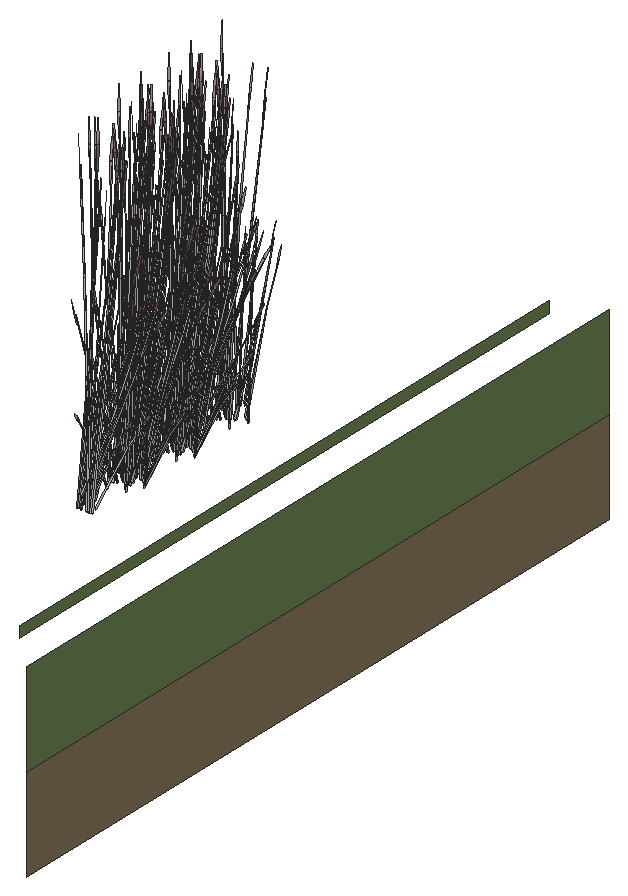
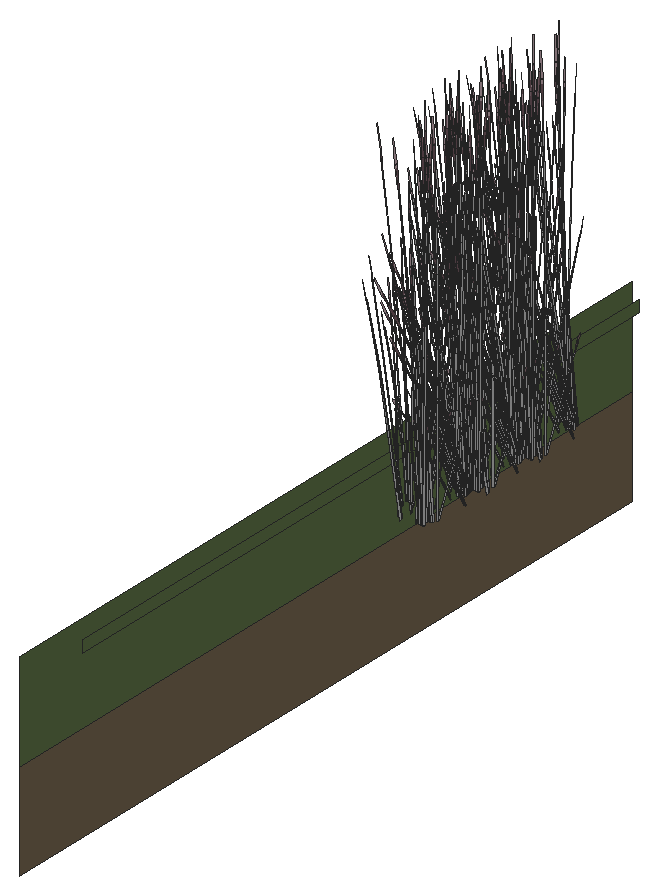
# SketchUp Ruby script. Lengths in inches.
U = 1.inch
M = Sketchup.active_model
def pt(a) = Geom::Point3d.new(a.map { |v| v * U })
def face(e, loops, mat)
  f = e.add_face(loops[0].map { |a| pt(a) })
  loops[1..].each { |l| e.add_face(l.map { |a| pt(a) }).erase! }
  f.material = f.back_material = mat if mat
  f
end
# faces: each face lists its corners as indices into pts; further lists are holes
def faces(e, pts, list, mat = nil) = list.each { |f| face(e, (f[0].is_a?(Array) ? f : [f]).map { |l| l.map { |i| pts[i] } }, mat) }
# xy, xz, yz: faces in a plane at the given z, y or x. An outline is a flat list of corners, or four numbers for a rectangle; further outlines are holes
def ring(l) = l.size == 4 ? [[l[0], l[1]], [l[2], l[1]], [l[2], l[3]], [l[0], l[3]]] : l.each_slice(2).to_a
def flat(e, list, mat, &to3) = list.each { |f| face(e, (f[0].is_a?(Array) ? f : [f]).map { |l| ring(l).map { |u, v| to3.(u, v) } }, mat) }
def xy(e, z, list, mat = nil) = flat(e, list, mat) { |x, y| [x, y, z] }
def xz(e, y, list, mat = nil) = flat(e, list, mat) { |x, z| [x, y, z] }
def yz(e, x, list, mat = nil) = flat(e, list, mat) { |y, z| [x, y, z] }
def lines(e, pts, list) = list.each { |a, b| e.add_line(pt(pts[a]), pt(pts[b])) }
# prism: a flat outline (further loops are holes) pulled along v
def prism(e, loops, v, mat = nil)
  f = face(e, loops, mat); d = Geom::Vector3d.new(v.map { |x| x * U })
  f.pushpull(f.normal.samedirection?(d) ? d.length : -d.length)
end
def box(e, o, s, mat = nil) = prism(e, [[o, [o[0] + s[0], o[1], o[2]], [o[0] + s[0], o[1] + s[1], o[2]], [o[0], o[1] + s[1], o[2]]]], [0, 0, s[2]], mat)
def at(x, y, z, deg = 0) = Geom::Transformation.translation(pt([x, y, z])) * Geom::Transformation.rotation(ORIGIN, Z_AXIS, deg.degrees)
def axes(o, x, y, z) = Geom::Transformation.new([*x, 0, *y, 0, *z, 0, *pt(o).to_a, 1])
def part(name) = M.definitions.add(name)
# library, detail: a bought-in or finely detailed component or shape, given as its bounding box
def library(name, o, s) = part(name).tap { |d| box(d.entities, o, s) }
def detail(e, o, s) = box(e.add_group.entities, o, s)
def put(e, d, t, mat = nil) = e.add_instance(d, t).tap { |i| i.material = mat if mat }
def group(e, t, mat = nil) = e.add_group.tap { |g| g.transformation = t; g.material = mat if mat }.entities
root = M.entities
M.materials.add("LightPink_Translucent").color = [144, 107, 117]
M.materials["LightPink_Translucent"].alpha = 0.75
M.materials.add("Plaster_03_1K").color = [121, 105, 83]
M.materials.add("Roofing_02_1K").color = [97, 118, 74]
M.materials.add("[_0053_Ivory_]").color = [200, 200, 200]
c1 = part("blade")
p = [[2.15,0.21,22],[0,0.17,0],[0.09,0.45,0],[2.18,0.31,22],[2.29,0.31,22],[0.38,0.45,0],
  [2.48,0.24,33],[2.49,0.24,33],[2.48,0.22,33]]
faces(c1.entities,p,[[0,1,2,3],[4,5,2,3],[6,3,4,7],[8,0,3,6]])
c2 = part("seeds")
p = [[0.3,-0.1,1.38],[-0.01,-0.03,1.59],[-0.01,-0.03,0.03],[0.14,-0.07,-0.07],[0.29,-0.03,3],[0.15,0.01,3.11]]
faces(c2.entities,p,[[0,1,2,3],[1,0,4,5]],"LightPink_Translucent")
c3 = part("blade with seeds")
put(c3.entities,c1,at(0,0,0))
put(c3.entities,c2,axes([2.4,0.25,30.99],[1.5799,-0.05474,1.17369],[-0.12525,1.92788,0.29478],[-0.07173,-0.02425,1.56792]))
yz(root,695.51,[[245.15,34,365.15,36]],"Roofing_02_1K")
yz(root,701.51,[[239.15,0,371.15,17]],"Plaster_03_1K")
yz(root,701.51,[[239.15,17,371.15,34]],"Roofing_02_1K")
put(root,c3,axes([680.55,278.33,35.86],[0.61229,0.28233,0],[-0.29468,0.58663,0],[0,0,1.74954]),"[_0053_Ivory_]")
put(root,c3,axes([681.82,278.08,38.63],[0.60713,0.01514,-0.71045],[-0.04078,0.63759,0.08574],[0.25721,0.06729,1.00501]),"[_0053_Ivory_]")
put(root,c3,axes([681.13,278.59,36.13],[0.56842,-0.31443,0.49651],[0.33976,0.56381,0],[-0.12946,0.07161,1.57504]),"[_0053_Ivory_]")
put(root,c3,axes([680.32,278.09,35.94],[0.26406,0.72244,-0.06012],[-0.7545,0.25315,0],[0.00922,0.02523,1.72173]),"[_0053_Ivory_]")
put(root,c3,axes([682.81,276.78,36.03],[0.75945,0,0],[0,0.70283,-0.51607],[0,0.16007,1.63711]),"[_0053_Ivory_]")
put(root,c3,axes([682.51,277.14,35.85],[-0.75908,-0.00503,-0.04976],[0,-0.70283,0.49943],[-0.02386,0.16,1.58352]),"[_0053_Ivory_]")
put(root,c3,axes([680.86,276.53,36.32],[0.68399,0.30005,-0.29095],[-0.32934,0.63331,-0.50002],[0.0215,0.15549,1.59708]),"[_0053_Ivory_]")
put(root,c3,axes([682.18,278.34,38.18],[0.34557,0.39372,-0.35414],[-0.39459,0.37271,0.4572],[0.20048,0.05671,0.87481]),"[_0053_Ivory_]")
put(root,c3,axes([682.35,277.25,35.68],[-0.42396,0.39235,-0.30978],[-0.42396,-0.39235,0.30978],[0,0.12637,1.38974]),"[_0053_Ivory_]")
put(root,c3,axes([680.79,277,35.86],[-0.29468,0.56664,-0.44739],[-0.61229,-0.27271,0.21531],[0,0.13062,1.43643]),"[_0053_Ivory_]")
put(root,c3,axes([680.81,278.63,35.98],[0.76036,0.2044,0.30756],[-0.19023,0.7306,-0.36492],[-0.12585,0.09144,1.64885]),"[_0053_Ivory_]")
put(root,c3,axes([682.64,277.26,35.67],[0,0.62885,-0.49651],[-0.67951,0,0],[0,0.14322,1.57504]),"[_0053_Ivory_]")
put(root,c3,axes([680.94,277.33,37.53],[-0.2256,-0.10835,1.71376],[0.46687,-0.45453,0.13857],[0.29098,0.20505,0.73262]),"[_0053_Ivory_]")
put(root,c3,axes([680.98,285.76,36.24],[-0.17264,0.12729,1.43002],[-0.51703,-0.22279,-0.30754],[0.09584,-0.27707,0.61141]),"[_0053_Ivory_]")
put(root,c3,axes([681.78,278.5625,36.42],[-0.34197,-0.18082,1.1486],[0.44156,-0.18372,0.84392],[0.1191,0.15563,0.25299]),"[_0053_Ivory_]")
put(root,c3,axes([679.7,285.07,35.15],[-0.10187,0.02266,1.76342],[-0.56336,-0.25503,-0.26939],[0.00945,-0.21273,0.30037]),"[_0053_Ivory_]")
put(root,c3,axes([681.4,286.7,38.63],[0.0158,-0.58168,-0.71045],[0.66548,0.03907,0.08574],[0.07023,-0.24643,1.00501]),"[_0053_Ivory_]")
put(root,c3,axes([681.87,279.24,35.15],[0.04425,-0.09079,1.76342],[0.55709,-0.26738,-0.26939],[0.16889,0.13839,0.30037]),"[_0053_Ivory_]")
put(root,c3,axes([680.25,285.77,38.18],[0.1831,-0.48359,-0.35414],[0.53419,0.14105,0.4572],[-0.04898,-0.1947,0.87481]),"[_0053_Ivory_]")
put(root,c3,axes([680.65,286.41,37.53],[-0.11309,0.21615,1.71376],[-0.47441,-0.44731,0.13857],[0.21402,-0.27879,0.73262]),"[_0053_Ivory_]")
put(root,c3,axes([681.14,277.17,35.75],[0.2227,0.57576,-0.69212],[-0.64151,0.20736,-0.18165],[0.02462,0.19497,1.52773]),"[_0053_Ivory_]")
put(root,c3,axes([681,278.8125,38.33],[0.59932,-0.14948,-0.51099],[0.10484,0.56611,-0.3958],[0.16097,0.16223,0.97773]),"[_0053_Ivory_]")
put(root,c3,axes([680.35,284.74,36.42],[0.07791,0.3667,1.1486],[-0.43222,-0.2031,0.84392],[0.04651,-0.18776,0.25299]),"[_0053_Ivory_]")
put(root,c3,axes([681.27,286.51,38.33],[-0.43478,-0.42253,-0.51099],[0.45929,-0.37004,-0.3958],[0.06615,-0.21468,0.97773]),"[_0053_Ivory_]")
put(root,c3,axes([681.83,279.39,36.32],[-0.38947,-0.01972,1.0506],[0.25721,-0.41888,0.58006],[0.15386,0.14882,0.8241]),"[_0053_Ivory_]")
put(root,c3,axes([681.68,286.35,38.18],[0.41095,-0.33109,-0.35414],[0.38901,0.37805,0.4572],[0.05919,-0.19208,0.87481]),"[_0053_Ivory_]")
put(root,c3,axes([680.56,278.37,36.24],[0.01072,-0.20846,1.43002],[0.51218,-0.23285,-0.30754],[0.15811,0.2495,0.61141]),"[_0053_Ivory_]")
put(root,c3,axes([679.27,279.22,35.15],[0.09829,-0.03422,1.76342],[0.59126,0.18834,-0.26939],[0.01729,0.21228,0.30037]),"[_0053_Ivory_]")
put(root,c3,axes([682.19,286.15,35.15],[-0.0909,-0.04954,1.76342],[-0.2335,-0.55347,-0.26939],[0.15752,-0.1502,0.30037]),"[_0053_Ivory_]")
put(root,c3,axes([679.67,279.08,38.33],[0.59704,0.15764,-0.51099],[-0.20464,0.54049,-0.3958],[0.05475,0.21761,0.97773]),"[_0053_Ivory_]")
put(root,c3,axes([680.01,277.96,37.53],[-0.13883,-0.2019,1.71376],[0.64153,-0.16998,0.13857],[0.14499,0.31697,0.73262]),"[_0053_Ivory_]")
put(root,c3,axes([679.4,279.41,38.18],[-0.1831,0.48359,-0.35414],[-0.53419,-0.14105,0.4572],[0.04898,0.1947,0.87481]),"[_0053_Ivory_]")
put(root,c3,axes([682.1875,287.71,38.63],[0.31725,-0.49618,-0.71045],[0.55593,0.35263,0.08574],[0.18942,-0.17977,1.00501]),"[_0053_Ivory_]")
put(root,c3,axes([678.76,286.27,36.03],[-0.37973,-0.63014,0],[0.6353,-0.35142,-0.51607],[0.14469,-0.08004,1.63711]),"[_0053_Ivory_]")
put(root,c3,axes([682.17,287.48,38.33],[-0.15602,-0.5742,-0.51099],[0.59087,-0.10045,-0.3958],[0.16933,-0.15423,0.97773]),"[_0053_Ivory_]")
put(root,c3,axes([679.46,278.97,38.63],[0.28988,0.51132,-0.71045],[-0.59671,0.28496,0.08574],[0.06778,0.24706,1.00501]),"[_0053_Ivory_]")
put(root,c3,axes([679.27,286.17,35.67],[0.56842,-0.31443,-0.49651],[0.33976,0.56381,0],[0.12946,-0.07161,1.57504]),"[_0053_Ivory_]")
put(root,c3,axes([682.65,287.26,36.24],[-0.21697,-0.01863,1.43002],[-0.22228,-0.49966,-0.30754],[0.26655,-0.14135,0.61141]),"[_0053_Ivory_]")
put(root,c3,axes([679.95,287.46,35.71],[0.40909,-0.47266,-0.62353],[0.50819,0.4286,-0.16365],[0.16393,-0.11791,1.37633]),"[_0053_Ivory_]")
put(root,c3,axes([682.9,286.34,36.42],[-0.2023,0.32011,1.1486],[-0.17388,-0.43009,0.84392],[0.16708,-0.10777,0.25299]),"[_0053_Ivory_]")
put(root,c3,axes([682.61,287.54,38.18],[0.52868,-0.08987,-0.35414],[0.1396,0.51376,0.4572],[0.1515,-0.13799,0.87481]),"[_0053_Ivory_]")
put(root,c3,axes([679.24,288.29,35.86],[0.29468,-0.56664,-0.44739],[0.61229,0.27271,0.21531],[0,-0.13062,1.43643]),"[_0053_Ivory_]")
put(root,c3,axes([679.5,288.01,36.32],[-0.07077,-0.71755,-0.29095],[0.73712,-0.04339,-0.50002],[0.1298,-0.09558,1.59708]),"[_0053_Ivory_]")
put(root,c3,axes([679.41,286.42,35.68],[0.56663,0.1556,-0.30978],[-0.14267,0.54795,0.30978],[0.11423,-0.06319,1.38974]),"[_0053_Ivory_]")
put(root,c3,axes([679.6,288.57,36.09],[0.68433,0.30479,0.24065],[-0.32934,0.63331,0.50002],[0,-0.14599,1.60543]),"[_0053_Ivory_]")
put(root,c3,axes([679.38,288.14,36.37],[-0.65953,0.03882,0.44739],[-0.05964,-0.64439,-0.21531],[0.11807,-0.06531,1.43643]),"[_0053_Ivory_]")
put(root,c3,axes([682.45,288.75,38.33],[0.16454,-0.57202,-0.51099],[0.56413,0.19607,-0.3958],[0.22713,-0.05245,0.97773]),"[_0053_Ivory_]")
put(root,c3,axes([681.55,286.43,36.03],[0.37973,-0.63014,0],[0.6353,0.35142,-0.51607],[0.14469,0.08004,1.63711]),"[_0053_Ivory_]")
put(root,c3,axes([679.36,288.375,36.01],[0.26406,0.70318,0.45755],[-0.7545,0.24452,0.17955],[0.00922,-0.12921,1.58856]),"[_0053_Ivory_]")
put(root,c3,axes([683.05,288.92,35.64],[-0.39118,0.07547,1.41583],[-0.06226,-0.6007,0.08104],[0.27398,-0.09092,0.80566]),"[_0053_Ivory_]")
put(root,c3,axes([683.76,288.38,35.91],[-0.37654,-0.40212,-0.06488],[0.4124,-0.36845,-0.29416],[0.11685,-0.02594,0.97024]),"[_0053_Ivory_]")
put(root,c3,axes([680.31,288.4375,35.86],[0,-0.72763,0],[0.75945,0,0],[0,0,1.79456]),"[_0053_Ivory_]")
put(root,c3,axes([681.23,286.75,36.13],[-0.56842,-0.31443,0.49651],[0.33976,-0.56381,0],[0.12946,0.07161,1.57504]),"[_0053_Ivory_]")
put(root,c3,axes([682.34,288.96,38.63],[0.53369,-0.27773,-0.71045],[0.29743,0.5717,0.08574],[0.25786,-0.06494,1.00501]),"[_0053_Ivory_]")
put(root,c3,axes([679.95,287.98,36.01],[-0.50358,0.57069,0.45755],[-0.59827,-0.50377,0.17955],[0.1214,-0.05695,1.58856]),"[_0053_Ivory_]")
put(root,c3,axes([679.07,287.04,36.13],[-0.17545,0.62497,0.17642],[-0.64204,-0.17686,0.35086],[0.11091,-0.00304,1.60407]),"[_0053_Ivory_]")
put(root,c3,axes([678.81,287.54,35.25],[-0.59782,0.25177,1.28929],[-0.19028,-0.72239,0.50096],[0.36709,0.01202,1.46642]),"[_0053_Ivory_]")
put(root,c3,axes([680.41,287.73,36.27],[0.11717,-0.56122,0.1448],[0.57245,0.09742,-0.41347],[0.10418,0.05763,1.26744]),"[_0053_Ivory_]")
put(root,c3,axes([683.48,288.52,35.15],[-0.03174,-0.09547,1.76342],[0.22015,-0.55846,-0.26939],[0.22208,-0.00803,0.30037]),"[_0053_Ivory_]")
put(root,c3,axes([680.17,287.88,36.37],[-0.36485,-0.52782,0.44739],[0.55265,-0.37168,-0.21531],[0.11807,0.06531,1.43643]),"[_0053_Ivory_]")
put(root,c3,axes([680.35,287.91,36.32],[0.61322,-0.4175,-0.29095],[0.40778,0.58992,-0.50002],[0.1513,0.05991,1.59708]),"[_0053_Ivory_]")
put(root,c3,axes([682.79,289.02,38.18],[0.50475,0.17543,-0.35414],[-0.14722,0.5118,0.4572],[0.20322,-0.04693,0.87481]),"[_0053_Ivory_]")
put(root,c3,axes([681.9,286.8,35.67],[0.56842,0.31443,-0.49651],[-0.33976,0.56381,0],[0.12946,0.07161,1.57504]),"[_0053_Ivory_]")
put(root,c3,axes([680.82,288.6,35.86],[0.67951,0,0],[0,0.65103,0],[0,0,1.78407]),"[_0053_Ivory_]")
put(root,c3,axes([681.01,287.07,36.13],[-0.65264,0.16691,0.17642],[-0.16115,-0.62115,0.35086],[0.05821,0.0905,1.60407]),"[_0053_Ivory_]")
put(root,c3,axes([681.42,288.38,37.53],[-0.25192,0.01424,1.71376],[0.16712,-0.61729,0.13857],[0.35901,0.03818,0.73262]),"[_0053_Ivory_]")
put(root,c3,axes([681.74,287.04,35.68],[0.14267,0.54795,-0.30978],[-0.56663,0.1556,0.30978],[0.11423,0.06319,1.38974]),"[_0053_Ivory_]")
put(root,c3,axes([680.6,288.27,36.03],[-0.76764,-0.13249,0.49198],[0.15622,-0.74829,0.19306],[0.11218,0.07226,1.70813]),"[_0053_Ivory_]")
put(root,c3,axes([679.99,290.11,35.86],[-0.19817,-0.54216,0],[0.56587,-0.18986,0],[0,0,1.54371]),"[_0053_Ivory_]")
put(root,c3,axes([680.73,290.04,35.84],[0.63764,-0.21337,-0.19198],[0.22406,0.61462,0.00008],[0.07038,-0.02358,1.73897]),"[_0053_Ivory_]")
put(root,c3,axes([680.81,288.88,35.87],[0.42396,0.40619,0],[-0.42396,0.40619,0],[0,0,1.69266]),"[_0053_Ivory_]")
put(root,c3,axes([681.95,288.7,36.13],[-0.47719,-0.45806,0.17642],[0.48088,-0.44429,0.35086],[-0.0527,0.09355,1.60407]),"[_0053_Ivory_]")
put(root,c3,axes([681.07,288.01,35.71],[0.63179,0.1031,-0.62353],[-0.13332,0.63596,-0.16365],[0.18854,0.07706,1.37633]),"[_0053_Ivory_]")
put(root,c3,axes([683.86,289.12,36.42],[-0.37526,0.10382,1.1486],[0.17664,-0.42906,0.84392],[0.19907,0.02936,0.25299]),"[_0053_Ivory_]")
put(root,c3,axes([680.8,288.4,36.37],[0.29468,-0.56664,0.44739],[0.61229,0.27271,-0.21531],[0,0.13062,1.43643]),"[_0053_Ivory_]")
put(root,c3,axes([680.6875,288.73,35.95],[0,0.72727,-0.05637],[-0.75945,0,0],[0,0.02286,1.79368]),"[_0053_Ivory_]")
put(root,c3,axes([680.74,288.21,35.86],[0.36485,0.52782,-0.44739],[-0.55265,0.37168,0.21531],[0.11807,0.06531,1.43643]),"[_0053_Ivory_]")
put(root,c3,axes([683.21,290.44,37.58],[-0.11624,-0.52862,-0.03492],[0.54943,-0.12153,-0.15832],[0.11473,0.03351,0.52218]),"[_0053_Ivory_]")
put(root,c3,axes([682.35,288.72,36.13],[0,-0.62885,0.49651],[0.67951,0,0],[0,0.14322,1.57504]),"[_0053_Ivory_]")
put(root,c3,axes([681.06,288.53,36.27],[0.56587,-0.18339,0.1448],[0.19817,0.52368,-0.41347],[0,0.11525,1.26744]),"[_0053_Ivory_]")
put(root,c3,axes([683.16,289.81,36.24],[-0.14627,-0.15466,1.43002],[0.19032,-0.51164,-0.30754],[0.29594,0.06931,0.61141]),"[_0053_Ivory_]")
put(root,c3,axes([680.55,290.37,35.86],[0.61229,0.28233,0],[-0.29468,0.58663,0],[0,0,1.74954]),"[_0053_Ivory_]")
put(root,c3,axes([681.82,290.12,38.63],[0.60713,0.01514,-0.71045],[-0.04078,0.63759,0.08574],[0.25721,0.06729,1.00501]),"[_0053_Ivory_]")
put(root,c3,axes([681.13,290.63,36.13],[0.56842,-0.31443,0.49651],[0.33976,0.56381,0],[-0.12946,0.07161,1.57504]),"[_0053_Ivory_]")
put(root,c3,axes([680.32,290.13,35.94],[0.26406,0.72244,-0.06012],[-0.7545,0.25315,0],[0.00922,0.02523,1.72173]),"[_0053_Ivory_]")
put(root,c3,axes([682.81,288.83,36.03],[0.75945,0,0],[0,0.70283,-0.51607],[0,0.16007,1.63711]),"[_0053_Ivory_]")
put(root,c3,axes([682.51,289.1875,35.85],[-0.75908,-0.00503,-0.04976],[0,-0.70283,0.49943],[-0.02386,0.16,1.58352]),"[_0053_Ivory_]")
put(root,c3,axes([680.86,288.57,36.32],[0.68399,0.30005,-0.29095],[-0.32934,0.63331,-0.50002],[0.0215,0.15549,1.59708]),"[_0053_Ivory_]")
put(root,c3,axes([682.18,290.38,38.18],[0.34557,0.39372,-0.35414],[-0.39459,0.37271,0.4572],[0.20048,0.05671,0.87481]),"[_0053_Ivory_]")
put(root,c3,axes([682.35,289.29,35.68],[-0.42396,0.39235,-0.30978],[-0.42396,-0.39235,0.30978],[0,0.12637,1.38974]),"[_0053_Ivory_]")
put(root,c3,axes([680.79,289.05,35.86],[-0.29468,0.56664,-0.44739],[-0.61229,-0.27271,0.21531],[0,0.13062,1.43643]),"[_0053_Ivory_]")
put(root,c3,axes([680.98,297.125,36.24],[-0.17264,0.12729,1.43002],[-0.51703,-0.22279,-0.30754],[0.09584,-0.27707,0.61141]),"[_0053_Ivory_]")
put(root,c3,axes([679.7,296.43,35.15],[-0.10187,0.02266,1.76342],[-0.56336,-0.25503,-0.26939],[0.00945,-0.21273,0.30037]),"[_0053_Ivory_]")
put(root,c3,axes([680.81,290.67,35.98],[0.76036,0.2044,0.30756],[-0.19023,0.7306,-0.36492],[-0.12585,0.09144,1.64885]),"[_0053_Ivory_]")
put(root,c3,axes([681.4,298.07,38.63],[0.0158,-0.58168,-0.71045],[0.66548,0.03907,0.08574],[0.07023,-0.24643,1.00501]),"[_0053_Ivory_]")
put(root,c3,axes([682.64,289.3,35.67],[0,0.62885,-0.49651],[-0.67951,0,0],[0,0.14322,1.57504]),"[_0053_Ivory_]")
put(root,c3,axes([680.94,289.37,37.53],[-0.2256,-0.10835,1.71376],[0.46687,-0.45453,0.13857],[0.29098,0.20505,0.73262]),"[_0053_Ivory_]")
put(root,c3,axes([680.25,297.13,38.18],[0.1831,-0.48359,-0.35414],[0.53419,0.14105,0.4572],[-0.04898,-0.1947,0.87481]),"[_0053_Ivory_]")
put(root,c3,axes([680.65,297.77,37.53],[-0.11309,0.21615,1.71376],[-0.47441,-0.44731,0.13857],[0.21402,-0.27879,0.73262]),"[_0053_Ivory_]")
put(root,c3,axes([681.78,290.61,36.42],[-0.34197,-0.18082,1.1486],[0.44156,-0.18372,0.84392],[0.1191,0.15563,0.25299]),"[_0053_Ivory_]")
put(root,c3,axes([680.35,296.11,36.42],[0.07791,0.3667,1.1486],[-0.43222,-0.2031,0.84392],[0.04651,-0.18776,0.25299]),"[_0053_Ivory_]")
put(root,c3,axes([681.27,297.875,38.33],[-0.43478,-0.42253,-0.51099],[0.45929,-0.37004,-0.3958],[0.06615,-0.21468,0.97773]),"[_0053_Ivory_]")
put(root,c3,axes([681.87,291.28,35.15],[0.04425,-0.09079,1.76342],[0.55709,-0.26738,-0.26939],[0.16889,0.13839,0.30037]),"[_0053_Ivory_]")
put(root,c3,axes([681.14,289.22,35.75],[0.2227,0.57576,-0.69212],[-0.64151,0.20736,-0.18165],[0.02462,0.19497,1.52773]),"[_0053_Ivory_]")
put(root,c3,axes([681,290.86,38.33],[0.59932,-0.14948,-0.51099],[0.10484,0.56611,-0.3958],[0.16097,0.16223,0.97773]),"[_0053_Ivory_]")
put(root,c3,axes([681.68,297.72,38.18],[0.41095,-0.33109,-0.35414],[0.38901,0.37805,0.4572],[0.05919,-0.19208,0.87481]),"[_0053_Ivory_]")
put(root,c3,axes([681.83,291.43,36.32],[-0.38947,-0.01972,1.0506],[0.25721,-0.41888,0.58006],[0.15386,0.14882,0.8241]),"[_0053_Ivory_]")
put(root,c3,axes([680.56,290.41,36.24],[0.01072,-0.20846,1.43002],[0.51218,-0.23285,-0.30754],[0.15811,0.2495,0.61141]),"[_0053_Ivory_]")
put(root,c3,axes([682.19,297.52,35.15],[-0.0909,-0.04954,1.76342],[-0.2335,-0.55347,-0.26939],[0.15752,-0.1502,0.30037]),"[_0053_Ivory_]")
put(root,c3,axes([679.27,291.26,35.15],[0.09829,-0.03422,1.76342],[0.59126,0.18834,-0.26939],[0.01729,0.21228,0.30037]),"[_0053_Ivory_]")
put(root,c3,axes([682.1875,299.08,38.63],[0.31725,-0.49618,-0.71045],[0.55593,0.35263,0.08574],[0.18942,-0.17977,1.00501]),"[_0053_Ivory_]")
put(root,c3,axes([678.76,297.63,36.03],[-0.37973,-0.63014,0],[0.6353,-0.35142,-0.51607],[0.14469,-0.08004,1.63711]),"[_0053_Ivory_]")
put(root,c3,axes([682.17,298.85,38.33],[-0.15602,-0.5742,-0.51099],[0.59087,-0.10045,-0.3958],[0.16933,-0.15423,0.97773]),"[_0053_Ivory_]")
put(root,c3,axes([679.67,291.12,38.33],[0.59704,0.15764,-0.51099],[-0.20464,0.54049,-0.3958],[0.05475,0.21761,0.97773]),"[_0053_Ivory_]")
put(root,c3,axes([680.01,290,37.53],[-0.13883,-0.2019,1.71376],[0.64153,-0.16998,0.13857],[0.14499,0.31697,0.73262]),"[_0053_Ivory_]")
put(root,c3,axes([679.4,291.45,38.18],[-0.1831,0.48359,-0.35414],[-0.53419,-0.14105,0.4572],[0.04898,0.1947,0.87481]),"[_0053_Ivory_]")
put(root,c3,axes([679.27,297.54,35.67],[0.56842,-0.31443,-0.49651],[0.33976,0.56381,0],[0.12946,-0.07161,1.57504]),"[_0053_Ivory_]")
put(root,c3,axes([682.65,298.625,36.24],[-0.21697,-0.01863,1.43002],[-0.22228,-0.49966,-0.30754],[0.26655,-0.14135,0.61141]),"[_0053_Ivory_]")
put(root,c3,axes([679.95,298.83,35.71],[0.40909,-0.47266,-0.62353],[0.50819,0.4286,-0.16365],[0.16393,-0.11791,1.37633]),"[_0053_Ivory_]")
put(root,c3,axes([682.9,297.7,36.42],[-0.2023,0.32011,1.1486],[-0.17388,-0.43009,0.84392],[0.16708,-0.10777,0.25299]),"[_0053_Ivory_]")
put(root,c3,axes([679.46,291.02,38.63],[0.28988,0.51132,-0.71045],[-0.59671,0.28496,0.08574],[0.06778,0.24706,1.00501]),"[_0053_Ivory_]")
put(root,c3,axes([682.61,298.91,38.18],[0.52868,-0.08987,-0.35414],[0.1396,0.51376,0.4572],[0.1515,-0.13799,0.87481]),"[_0053_Ivory_]")
put(root,c3,axes([679.24,299.66,35.86],[0.29468,-0.56664,-0.44739],[0.61229,0.27271,0.21531],[0,-0.13062,1.43643]),"[_0053_Ivory_]")
put(root,c3,axes([679.5,299.375,36.32],[-0.07077,-0.71755,-0.29095],[0.73712,-0.04339,-0.50002],[0.1298,-0.09558,1.59708]),"[_0053_Ivory_]")
put(root,c3,axes([679.41,297.79,35.68],[0.56663,0.1556,-0.30978],[-0.14267,0.54795,0.30978],[0.11423,-0.06319,1.38974]),"[_0053_Ivory_]")
put(root,c3,axes([679.6,299.9375,36.09],[0.68433,0.30479,0.24065],[-0.32934,0.63331,0.50002],[0,-0.14599,1.60543]),"[_0053_Ivory_]")
put(root,c3,axes([679.38,299.51,36.37],[-0.65953,0.03882,0.44739],[-0.05964,-0.64439,-0.21531],[0.11807,-0.06531,1.43643]),"[_0053_Ivory_]")
put(root,c3,axes([682.45,300.12,38.33],[0.16454,-0.57202,-0.51099],[0.56413,0.19607,-0.3958],[0.22713,-0.05245,0.97773]),"[_0053_Ivory_]")
put(root,c3,axes([681.55,297.79,36.03],[0.37973,-0.63014,0],[0.6353,0.35142,-0.51607],[0.14469,0.08004,1.63711]),"[_0053_Ivory_]")
put(root,c3,axes([679.36,299.74,36.01],[0.26406,0.70318,0.45755],[-0.7545,0.24452,0.17955],[0.00922,-0.12921,1.58856]),"[_0053_Ivory_]")
put(root,c3,axes([683.05,300.28,35.64],[-0.39118,0.07547,1.41583],[-0.06226,-0.6007,0.08104],[0.27398,-0.09092,0.80566]),"[_0053_Ivory_]")
put(root,c3,axes([683.76,299.75,35.91],[-0.37654,-0.40212,-0.06488],[0.4124,-0.36845,-0.29416],[0.11685,-0.02594,0.97024]),"[_0053_Ivory_]")
put(root,c3,axes([680.31,299.8,35.86],[0,-0.72763,0],[0.75945,0,0],[0,0,1.79456]),"[_0053_Ivory_]")
put(root,c3,axes([681.23,298.12,36.13],[-0.56842,-0.31443,0.49651],[0.33976,-0.56381,0],[0.12946,0.07161,1.57504]),"[_0053_Ivory_]")
put(root,c3,axes([682.34,300.33,38.63],[0.53369,-0.27773,-0.71045],[0.29743,0.5717,0.08574],[0.25786,-0.06494,1.00501]),"[_0053_Ivory_]")
put(root,c3,axes([679.95,299.35,36.01],[-0.50358,0.57069,0.45755],[-0.59827,-0.50377,0.17955],[0.1214,-0.05695,1.58856]),"[_0053_Ivory_]")
put(root,c3,axes([679.07,298.41,36.13],[-0.17545,0.62497,0.17642],[-0.64204,-0.17686,0.35086],[0.11091,-0.00304,1.60407]),"[_0053_Ivory_]")
put(root,c3,axes([678.81,298.91,35.25],[-0.59782,0.25177,1.28929],[-0.19028,-0.72239,0.50096],[0.36709,0.01202,1.46642]),"[_0053_Ivory_]")
put(root,c3,axes([680.41,299.1,36.27],[0.11717,-0.56122,0.1448],[0.57245,0.09742,-0.41347],[0.10418,0.05763,1.26744]),"[_0053_Ivory_]")
put(root,c3,axes([683.48,299.89,35.15],[-0.03174,-0.09547,1.76342],[0.22015,-0.55846,-0.26939],[0.22208,-0.00803,0.30037]),"[_0053_Ivory_]")
put(root,c3,axes([680.17,299.25,36.37],[-0.36485,-0.52782,0.44739],[0.55265,-0.37168,-0.21531],[0.11807,0.06531,1.43643]),"[_0053_Ivory_]")
put(root,c3,axes([680.35,299.28,36.32],[0.61322,-0.4175,-0.29095],[0.40778,0.58992,-0.50002],[0.1513,0.05991,1.59708]),"[_0053_Ivory_]")
put(root,c3,axes([682.79,300.38,38.18],[0.50475,0.17543,-0.35414],[-0.14722,0.5118,0.4572],[0.20322,-0.04693,0.87481]),"[_0053_Ivory_]")
put(root,c3,axes([681.9,298.17,35.67],[0.56842,0.31443,-0.49651],[-0.33976,0.56381,0],[0.12946,0.07161,1.57504]),"[_0053_Ivory_]")
put(root,c3,axes([680.82,299.97,35.86],[0.67951,0,0],[0,0.65103,0],[0,0,1.78407]),"[_0053_Ivory_]")
put(root,c3,axes([681.01,298.44,36.13],[-0.65264,0.16691,0.17642],[-0.16115,-0.62115,0.35086],[0.05821,0.0905,1.60407]),"[_0053_Ivory_]")
put(root,c3,axes([681.42,299.75,37.53],[-0.25192,0.01424,1.71376],[0.16712,-0.61729,0.13857],[0.35901,0.03818,0.73262]),"[_0053_Ivory_]")
put(root,c3,axes([681.74,298.41,35.68],[0.14267,0.54795,-0.30978],[-0.56663,0.1556,0.30978],[0.11423,0.06319,1.38974]),"[_0053_Ivory_]")
put(root,c3,axes([680.6,299.63,36.03],[-0.76764,-0.13249,0.49198],[0.15622,-0.74829,0.19306],[0.11218,0.07226,1.70813]),"[_0053_Ivory_]")
put(root,c3,axes([679.99,301.48,35.86],[-0.19817,-0.54216,0],[0.56587,-0.18986,0],[0,0,1.54371]),"[_0053_Ivory_]")
put(root,c3,axes([680.73,301.41,35.84],[0.63764,-0.21337,-0.19198],[0.22406,0.61462,0.00008],[0.07038,-0.02358,1.73897]),"[_0053_Ivory_]")
put(root,c3,axes([680.81,300.25,35.87],[0.42396,0.40619,0],[-0.42396,0.40619,0],[0,0,1.69266]),"[_0053_Ivory_]")
put(root,c3,axes([681.95,300.07,36.13],[-0.47719,-0.45806,0.17642],[0.48088,-0.44429,0.35086],[-0.0527,0.09355,1.60407]),"[_0053_Ivory_]")
put(root,c3,axes([681.07,299.375,35.71],[0.63179,0.1031,-0.62353],[-0.13332,0.63596,-0.16365],[0.18854,0.07706,1.37633]),"[_0053_Ivory_]")
put(root,c3,axes([683.86,300.49,36.42],[-0.37526,0.10382,1.1486],[0.17664,-0.42906,0.84392],[0.19907,0.02936,0.25299]),"[_0053_Ivory_]")
put(root,c3,axes([680.8,299.77,36.37],[0.29468,-0.56664,0.44739],[0.61229,0.27271,-0.21531],[0,0.13062,1.43643]),"[_0053_Ivory_]")
put(root,c3,axes([680.6875,300.09,35.95],[0,0.72727,-0.05637],[-0.75945,0,0],[0,0.02286,1.79368]),"[_0053_Ivory_]")
put(root,c3,axes([680.74,299.58,35.86],[0.36485,0.52782,-0.44739],[-0.55265,0.37168,0.21531],[0.11807,0.06531,1.43643]),"[_0053_Ivory_]")
put(root,c3,axes([683.21,301.81,37.58],[-0.11624,-0.52862,-0.03492],[0.54943,-0.12153,-0.15832],[0.11473,0.03351,0.52218]),"[_0053_Ivory_]")
put(root,c3,axes([682.35,300.09,36.13],[0,-0.62885,0.49651],[0.67951,0,0],[0,0.14322,1.57504]),"[_0053_Ivory_]")
put(root,c3,axes([681.06,299.9,36.27],[0.56587,-0.18339,0.1448],[0.19817,0.52368,-0.41347],[0,0.11525,1.26744]),"[_0053_Ivory_]")
put(root,c3,axes([683.16,301.18,36.24],[-0.14627,-0.15466,1.43002],[0.19032,-0.51164,-0.30754],[0.29594,0.06931,0.61141]),"[_0053_Ivory_]")
put(root,c3,axes([680.55,301.74,35.86],[0.61229,0.28233,0],[-0.29468,0.58663,0],[0,0,1.74954]),"[_0053_Ivory_]")
put(root,c3,axes([681.82,301.49,38.63],[0.60713,0.01514,-0.71045],[-0.04078,0.63759,0.08574],[0.25721,0.06729,1.00501]),"[_0053_Ivory_]")
put(root,c3,axes([681.13,302,36.13],[0.56842,-0.31443,0.49651],[0.33976,0.56381,0],[-0.12946,0.07161,1.57504]),"[_0053_Ivory_]")
put(root,c3,axes([680.32,301.5,35.94],[0.26406,0.72244,-0.06012],[-0.7545,0.25315,0],[0.00922,0.02523,1.72173]),"[_0053_Ivory_]")
put(root,c3,axes([682.81,300.19,36.03],[0.75945,0,0],[0,0.70283,-0.51607],[0,0.16007,1.63711]),"[_0053_Ivory_]")
put(root,c3,axes([682.51,300.55,35.85],[-0.75908,-0.00503,-0.04976],[0,-0.70283,0.49943],[-0.02386,0.16,1.58352]),"[_0053_Ivory_]")
put(root,c3,axes([680.86,299.94,36.32],[0.68399,0.30005,-0.29095],[-0.32934,0.63331,-0.50002],[0.0215,0.15549,1.59708]),"[_0053_Ivory_]")
put(root,c3,axes([682.18,301.75,38.18],[0.34557,0.39372,-0.35414],[-0.39459,0.37271,0.4572],[0.20048,0.05671,0.87481]),"[_0053_Ivory_]")
put(root,c3,axes([682.35,300.66,35.68],[-0.42396,0.39235,-0.30978],[-0.42396,-0.39235,0.30978],[0,0.12637,1.38974]),"[_0053_Ivory_]")
put(root,c3,axes([680.79,300.41,35.86],[-0.29468,0.56664,-0.44739],[-0.61229,-0.27271,0.21531],[0,0.13062,1.43643]),"[_0053_Ivory_]")
put(root,c3,axes([680.81,302.04,35.98],[0.76036,0.2044,0.30756],[-0.19023,0.7306,-0.36492],[-0.12585,0.09144,1.64885]),"[_0053_Ivory_]")
put(root,c3,axes([682.64,300.67,35.67],[0,0.62885,-0.49651],[-0.67951,0,0],[0,0.14322,1.57504]),"[_0053_Ivory_]")
put(root,c3,axes([680.94,300.74,37.53],[-0.2256,-0.10835,1.71376],[0.46687,-0.45453,0.13857],[0.29098,0.20505,0.73262]),"[_0053_Ivory_]")
put(root,c3,axes([680.98,309.1,36.24],[-0.17264,0.12729,1.43002],[-0.51703,-0.22279,-0.30754],[0.09584,-0.27707,0.61141]),"[_0053_Ivory_]")
put(root,c3,axes([681.78,301.97,36.42],[-0.34197,-0.18082,1.1486],[0.44156,-0.18372,0.84392],[0.1191,0.15563,0.25299]),"[_0053_Ivory_]")
put(root,c3,axes([679.7,308.41,35.15],[-0.10187,0.02266,1.76342],[-0.56336,-0.25503,-0.26939],[0.00945,-0.21273,0.30037]),"[_0053_Ivory_]")
put(root,c3,axes([681.4,310.05,38.63],[0.0158,-0.58168,-0.71045],[0.66548,0.03907,0.08574],[0.07023,-0.24643,1.00501]),"[_0053_Ivory_]")
put(root,c3,axes([680.25,309.11,38.18],[0.1831,-0.48359,-0.35414],[0.53419,0.14105,0.4572],[-0.04898,-0.1947,0.87481]),"[_0053_Ivory_]")
put(root,c3,axes([680.65,309.75,37.53],[-0.11309,0.21615,1.71376],[-0.47441,-0.44731,0.13857],[0.21402,-0.27879,0.73262]),"[_0053_Ivory_]")
put(root,c3,axes([681.87,302.65,35.15],[0.04425,-0.09079,1.76342],[0.55709,-0.26738,-0.26939],[0.16889,0.13839,0.30037]),"[_0053_Ivory_]")
put(root,c3,axes([681.14,300.58,35.75],[0.2227,0.57576,-0.69212],[-0.64151,0.20736,-0.18165],[0.02462,0.19497,1.52773]),"[_0053_Ivory_]")
put(root,c3,axes([681,302.22,38.33],[0.59932,-0.14948,-0.51099],[0.10484,0.56611,-0.3958],[0.16097,0.16223,0.97773]),"[_0053_Ivory_]")
put(root,c3,axes([680.35,308.09,36.42],[0.07791,0.3667,1.1486],[-0.43222,-0.2031,0.84392],[0.04651,-0.18776,0.25299]),"[_0053_Ivory_]")
put(root,c3,axes([681.27,309.85,38.33],[-0.43478,-0.42253,-0.51099],[0.45929,-0.37004,-0.3958],[0.06615,-0.21468,0.97773]),"[_0053_Ivory_]")
put(root,c3,axes([681.83,302.8,36.32],[-0.38947,-0.01972,1.0506],[0.25721,-0.41888,0.58006],[0.15386,0.14882,0.8241]),"[_0053_Ivory_]")
put(root,c3,axes([681.68,309.7,38.18],[0.41095,-0.33109,-0.35414],[0.38901,0.37805,0.4572],[0.05919,-0.19208,0.87481]),"[_0053_Ivory_]")
put(root,c3,axes([680.56,301.78,36.24],[0.01072,-0.20846,1.43002],[0.51218,-0.23285,-0.30754],[0.15811,0.2495,0.61141]),"[_0053_Ivory_]")
put(root,c3,axes([679.27,302.625,35.15],[0.09829,-0.03422,1.76342],[0.59126,0.18834,-0.26939],[0.01729,0.21228,0.30037]),"[_0053_Ivory_]")
put(root,c3,axes([682.19,309.5,35.15],[-0.0909,-0.04954,1.76342],[-0.2335,-0.55347,-0.26939],[0.15752,-0.1502,0.30037]),"[_0053_Ivory_]")
put(root,c3,axes([679.67,302.49,38.33],[0.59704,0.15764,-0.51099],[-0.20464,0.54049,-0.3958],[0.05475,0.21761,0.97773]),"[_0053_Ivory_]")
put(root,c3,axes([680.01,301.37,37.53],[-0.13883,-0.2019,1.71376],[0.64153,-0.16998,0.13857],[0.14499,0.31697,0.73262]),"[_0053_Ivory_]")
put(root,c3,axes([679.4,302.82,38.18],[-0.1831,0.48359,-0.35414],[-0.53419,-0.14105,0.4572],[0.04898,0.1947,0.87481]),"[_0053_Ivory_]")
put(root,c3,axes([682.1875,311.06,38.63],[0.31725,-0.49618,-0.71045],[0.55593,0.35263,0.08574],[0.18942,-0.17977,1.00501]),"[_0053_Ivory_]")
put(root,c3,axes([678.76,309.61,36.03],[-0.37973,-0.63014,0],[0.6353,-0.35142,-0.51607],[0.14469,-0.08004,1.63711]),"[_0053_Ivory_]")
put(root,c3,axes([682.17,310.82,38.33],[-0.15602,-0.5742,-0.51099],[0.59087,-0.10045,-0.3958],[0.16933,-0.15423,0.97773]),"[_0053_Ivory_]")
put(root,c3,axes([679.46,302.38,38.63],[0.28988,0.51132,-0.71045],[-0.59671,0.28496,0.08574],[0.06778,0.24706,1.00501]),"[_0053_Ivory_]")
put(root,c3,axes([679.27,309.51,35.67],[0.56842,-0.31443,-0.49651],[0.33976,0.56381,0],[0.12946,-0.07161,1.57504]),"[_0053_Ivory_]")
put(root,c3,axes([682.65,310.6,36.24],[-0.21697,-0.01863,1.43002],[-0.22228,-0.49966,-0.30754],[0.26655,-0.14135,0.61141]),"[_0053_Ivory_]")
put(root,c3,axes([679.95,310.8,35.71],[0.40909,-0.47266,-0.62353],[0.50819,0.4286,-0.16365],[0.16393,-0.11791,1.37633]),"[_0053_Ivory_]")
put(root,c3,axes([682.9,309.68,36.42],[-0.2023,0.32011,1.1486],[-0.17388,-0.43009,0.84392],[0.16708,-0.10777,0.25299]),"[_0053_Ivory_]")
put(root,c3,axes([682.61,310.89,38.18],[0.52868,-0.08987,-0.35414],[0.1396,0.51376,0.4572],[0.1515,-0.13799,0.87481]),"[_0053_Ivory_]")
put(root,c3,axes([679.24,311.63,35.86],[0.29468,-0.56664,-0.44739],[0.61229,0.27271,0.21531],[0,-0.13062,1.43643]),"[_0053_Ivory_]")
put(root,c3,axes([679.5,311.35,36.32],[-0.07077,-0.71755,-0.29095],[0.73712,-0.04339,-0.50002],[0.1298,-0.09558,1.59708]),"[_0053_Ivory_]")
put(root,c3,axes([679.41,309.76,35.68],[0.56663,0.1556,-0.30978],[-0.14267,0.54795,0.30978],[0.11423,-0.06319,1.38974]),"[_0053_Ivory_]")
put(root,c3,axes([679.6,311.91,36.09],[0.68433,0.30479,0.24065],[-0.32934,0.63331,0.50002],[0,-0.14599,1.60543]),"[_0053_Ivory_]")
put(root,c3,axes([679.38,311.49,36.37],[-0.65953,0.03882,0.44739],[-0.05964,-0.64439,-0.21531],[0.11807,-0.06531,1.43643]),"[_0053_Ivory_]")
put(root,c3,axes([682.45,312.1,38.33],[0.16454,-0.57202,-0.51099],[0.56413,0.19607,-0.3958],[0.22713,-0.05245,0.97773]),"[_0053_Ivory_]")
put(root,c3,axes([681.55,309.77,36.03],[0.37973,-0.63014,0],[0.6353,0.35142,-0.51607],[0.14469,0.08004,1.63711]),"[_0053_Ivory_]")
put(root,c3,axes([679.36,311.72,36.01],[0.26406,0.70318,0.45755],[-0.7545,0.24452,0.17955],[0.00922,-0.12921,1.58856]),"[_0053_Ivory_]")
put(root,c3,axes([683.05,312.26,35.64],[-0.39118,0.07547,1.41583],[-0.06226,-0.6007,0.08104],[0.27398,-0.09092,0.80566]),"[_0053_Ivory_]")
put(root,c3,axes([683.76,311.73,35.91],[-0.37654,-0.40212,-0.06488],[0.4124,-0.36845,-0.29416],[0.11685,-0.02594,0.97024]),"[_0053_Ivory_]")
put(root,c3,axes([680.31,311.78,35.86],[0,-0.72763,0],[0.75945,0,0],[0,0,1.79456]),"[_0053_Ivory_]")
put(root,c3,axes([681.23,310.1,36.13],[-0.56842,-0.31443,0.49651],[0.33976,-0.56381,0],[0.12946,0.07161,1.57504]),"[_0053_Ivory_]")
